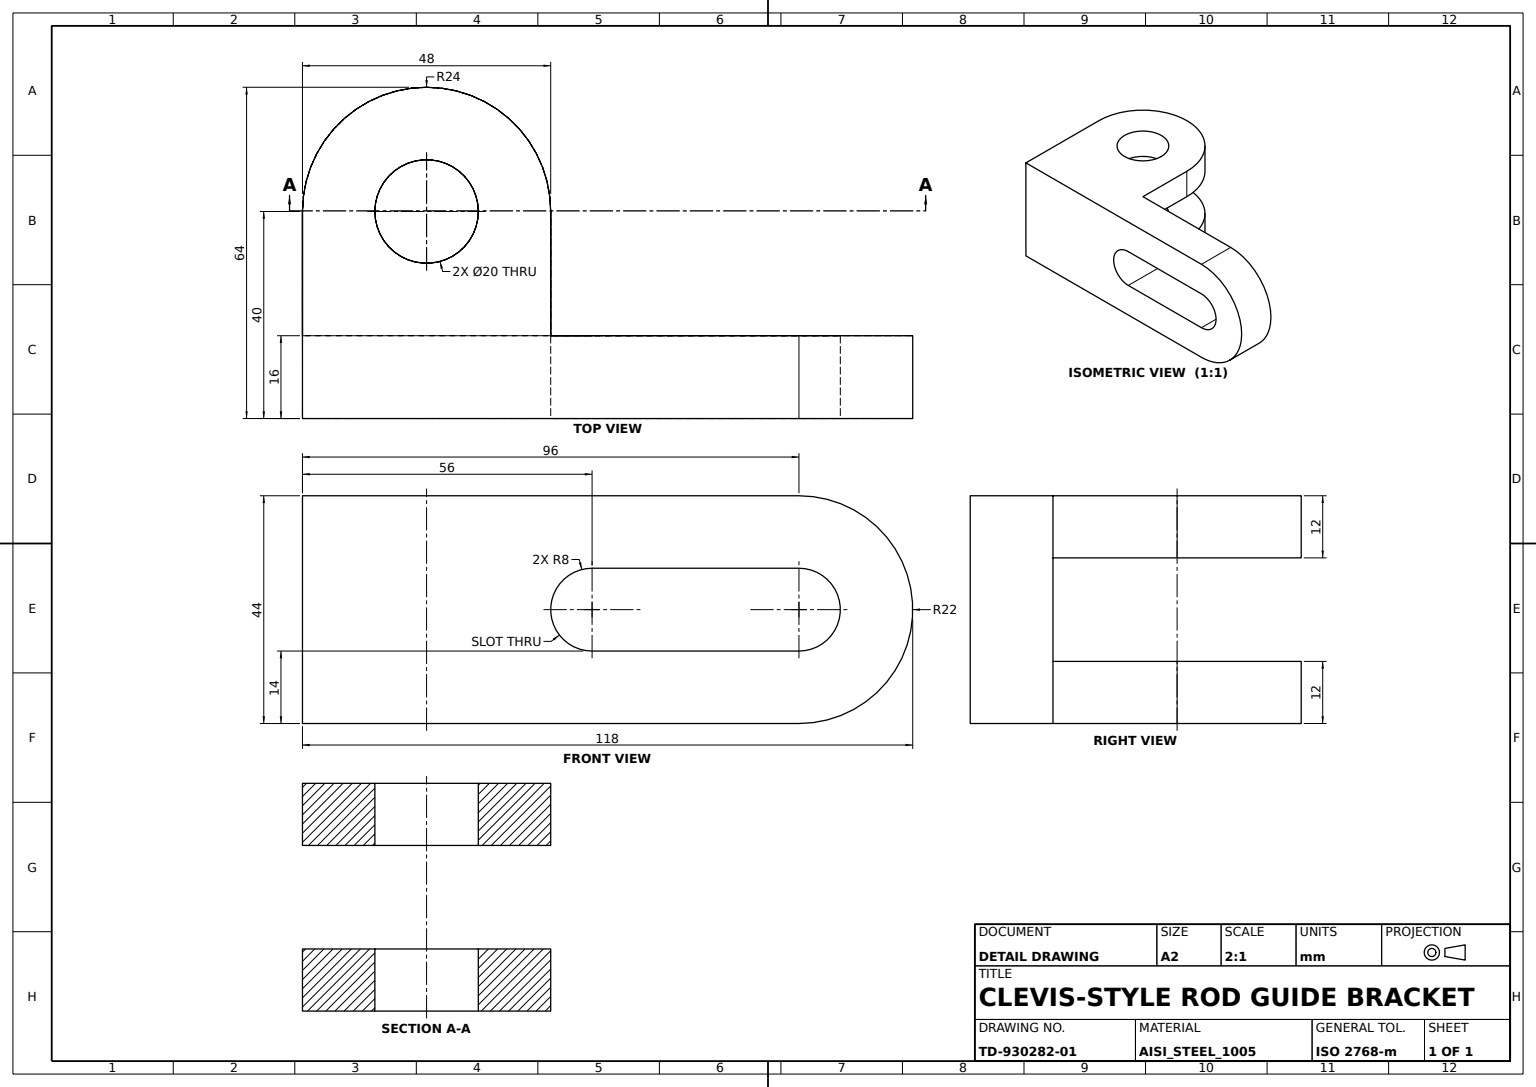
ISO-10303-21;
HEADER;
FILE_DESCRIPTION((''),'2;1');
FILE_NAME('','',(''),(''),'','','');
FILE_SCHEMA(('AUTOMOTIVE_DESIGN'));
ENDSEC;
DATA;
#1=APPLICATION_CONTEXT('');
#2=PRODUCT_CONTEXT('',#1,'mechanical');
#3=PRODUCT('','','',(#2));
#4=PRODUCT_DEFINITION_FORMATION('','',#3);
#5=PRODUCT_DEFINITION_CONTEXT('',#1,'design');
#6=PRODUCT_DEFINITION('','',#4,#5);
#7=PRODUCT_DEFINITION_SHAPE('','',#6);
#8=(LENGTH_UNIT()NAMED_UNIT(*)SI_UNIT(.MILLI.,.METRE.));
#9=(NAMED_UNIT(*)PLANE_ANGLE_UNIT()SI_UNIT($,.RADIAN.));
#10=(NAMED_UNIT(*)SI_UNIT($,.STERADIAN.)SOLID_ANGLE_UNIT());
#11=UNCERTAINTY_MEASURE_WITH_UNIT(LENGTH_MEASURE(0.005),#8,'distance_accuracy_value','');
#12=(GEOMETRIC_REPRESENTATION_CONTEXT(3)GLOBAL_UNCERTAINTY_ASSIGNED_CONTEXT((#11))GLOBAL_UNIT_ASSIGNED_CONTEXT((#8,#9,#10))REPRESENTATION_CONTEXT('',''));
#13=CARTESIAN_POINT('',(96.,16.,8.));
#14=VERTEX_POINT('',#13);
#15=CARTESIAN_POINT('',(96.,0.,8.));
#16=VERTEX_POINT('',#15);
#17=DIRECTION('',(0.,-1.,0.));
#18=VECTOR('',#17,1000.);
#19=LINE('',#13,#18);
#20=EDGE_CURVE('',#14,#16,#19,.T.);
#21=ORIENTED_EDGE('',*,*,#20,.F.);
#22=CARTESIAN_POINT('',(96.,16.,-8.));
#23=VERTEX_POINT('',#22);
#24=CARTESIAN_POINT('',(96.,16.,0.));
#25=DIRECTION('',(1.,0.,0.));
#26=AXIS2_PLACEMENT_3D('',#24,#17,#25);
#27=CIRCLE('',#26,8.);
#28=EDGE_CURVE('',#23,#14,#27,.T.);
#29=ORIENTED_EDGE('',*,*,#28,.F.);
#30=CARTESIAN_POINT('',(96.,0.,-8.));
#31=VERTEX_POINT('',#30);
#32=LINE('',#22,#18);
#33=EDGE_CURVE('',#23,#31,#32,.T.);
#34=ORIENTED_EDGE('',*,*,#33,.T.);
#35=CARTESIAN_POINT('',(96.,0.,0.));
#36=AXIS2_PLACEMENT_3D('',#35,#17,#25);
#37=CIRCLE('',#36,8.);
#38=EDGE_CURVE('',#31,#16,#37,.T.);
#39=ORIENTED_EDGE('',*,*,#38,.T.);
#40=EDGE_LOOP('',(#21,#29,#34,#39));
#41=FACE_BOUND('',#40,.T.);
#42=DIRECTION('',(0.,0.,-1.));
#43=AXIS2_PLACEMENT_3D('',#24,#17,#42);
#44=CYLINDRICAL_SURFACE('',#43,8.);
#45=ADVANCED_FACE('',(#41),#44,.F.);
#46=CARTESIAN_POINT('',(56.,16.,8.));
#47=VERTEX_POINT('',#46);
#48=DIRECTION('',(-1.,0.,0.));
#49=VECTOR('',#48,1000.);
#50=LINE('',#13,#49);
#51=EDGE_CURVE('',#14,#47,#50,.T.);
#52=ORIENTED_EDGE('',*,*,#51,.F.);
#53=ORIENTED_EDGE('',*,*,#20,.T.);
#54=CARTESIAN_POINT('',(56.,0.,8.));
#55=VERTEX_POINT('',#54);
#56=LINE('',#15,#49);
#57=EDGE_CURVE('',#16,#55,#56,.T.);
#58=ORIENTED_EDGE('',*,*,#57,.T.);
#59=LINE('',#46,#18);
#60=EDGE_CURVE('',#47,#55,#59,.T.);
#61=ORIENTED_EDGE('',*,*,#60,.F.);
#62=EDGE_LOOP('',(#52,#53,#58,#61));
#63=FACE_BOUND('',#62,.T.);
#64=DIRECTION('',(0.,0.,1.));
#65=AXIS2_PLACEMENT_3D('',#13,#64,#25);
#66=PLANE('',#65);
#67=ADVANCED_FACE('',(#63),#66,.F.);
#68=CARTESIAN_POINT('',(48.,40.,10.));
#69=VERTEX_POINT('',#68);
#70=CARTESIAN_POINT('',(48.,40.,22.));
#71=VERTEX_POINT('',#70);
#72=VECTOR('',#64,1000.);
#73=LINE('',#68,#72);
#74=EDGE_CURVE('',#69,#71,#73,.T.);
#75=ORIENTED_EDGE('',*,*,#74,.F.);
#76=CARTESIAN_POINT('',(0.,40.,10.));
#77=VERTEX_POINT('',#76);
#78=CARTESIAN_POINT('',(24.,40.,10.));
#79=AXIS2_PLACEMENT_3D('',#78,#64,#25);
#80=CIRCLE('',#79,24.);
#81=EDGE_CURVE('',#69,#77,#80,.T.);
#82=ORIENTED_EDGE('',*,*,#81,.T.);
#83=CARTESIAN_POINT('',(0.,40.,22.));
#84=VERTEX_POINT('',#83);
#85=LINE('',#76,#72);
#86=EDGE_CURVE('',#77,#84,#85,.T.);
#87=ORIENTED_EDGE('',*,*,#86,.T.);
#88=CARTESIAN_POINT('',(24.,40.,22.));
#89=AXIS2_PLACEMENT_3D('',#88,#64,#25);
#90=CIRCLE('',#89,24.);
#91=EDGE_CURVE('',#71,#84,#90,.T.);
#92=ORIENTED_EDGE('',*,*,#91,.F.);
#93=EDGE_LOOP('',(#75,#82,#87,#92));
#94=FACE_BOUND('',#93,.T.);
#95=CYLINDRICAL_SURFACE('',#79,24.);
#96=ADVANCED_FACE('',(#94),#95,.T.);
#97=ORIENTED_EDGE('',*,*,#60,.T.);
#98=CARTESIAN_POINT('',(56.,0.,-8.));
#99=VERTEX_POINT('',#98);
#100=CARTESIAN_POINT('',(56.,0.,0.));
#101=AXIS2_PLACEMENT_3D('',#100,#17,#25);
#102=CIRCLE('',#101,8.);
#103=EDGE_CURVE('',#55,#99,#102,.T.);
#104=ORIENTED_EDGE('',*,*,#103,.T.);
#105=CARTESIAN_POINT('',(56.,16.,-8.));
#106=VERTEX_POINT('',#105);
#107=LINE('',#105,#18);
#108=EDGE_CURVE('',#106,#99,#107,.T.);
#109=ORIENTED_EDGE('',*,*,#108,.F.);
#110=CARTESIAN_POINT('',(56.,16.,0.));
#111=AXIS2_PLACEMENT_3D('',#110,#17,#25);
#112=CIRCLE('',#111,8.);
#113=EDGE_CURVE('',#47,#106,#112,.T.);
#114=ORIENTED_EDGE('',*,*,#113,.F.);
#115=EDGE_LOOP('',(#97,#104,#109,#114));
#116=FACE_BOUND('',#115,.T.);
#117=AXIS2_PLACEMENT_3D('',#110,#17,#42);
#118=CYLINDRICAL_SURFACE('',#117,8.);
#119=ADVANCED_FACE('',(#116),#118,.F.);
#120=CARTESIAN_POINT('',(34.,40.,-22.));
#121=VERTEX_POINT('',#120);
#122=CARTESIAN_POINT('',(24.,40.,-22.));
#123=AXIS2_PLACEMENT_3D('',#122,#64,#25);
#124=CIRCLE('',#123,10.);
#125=EDGE_CURVE('',#121,#121,#124,.T.);
#126=ORIENTED_EDGE('',*,*,#125,.F.);
#127=EDGE_LOOP('',(#126));
#128=FACE_BOUND('',#127,.T.);
#129=CARTESIAN_POINT('',(34.,40.,-10.));
#130=VERTEX_POINT('',#129);
#131=CARTESIAN_POINT('',(24.,40.,-10.));
#132=AXIS2_PLACEMENT_3D('',#131,#64,#25);
#133=CIRCLE('',#132,10.);
#134=EDGE_CURVE('',#130,#130,#133,.T.);
#135=ORIENTED_EDGE('',*,*,#134,.T.);
#136=EDGE_LOOP('',(#135));
#137=FACE_BOUND('',#136,.T.);
#138=AXIS2_PLACEMENT_3D('',#131,#42,#48);
#139=CYLINDRICAL_SURFACE('',#138,10.);
#140=ADVANCED_FACE('',(#128,#137),#139,.F.);
#141=CARTESIAN_POINT('',(34.,40.,22.));
#142=VERTEX_POINT('',#141);
#143=CIRCLE('',#89,10.);
#144=EDGE_CURVE('',#142,#142,#143,.T.);
#145=ORIENTED_EDGE('',*,*,#144,.F.);
#146=EDGE_LOOP('',(#145));
#147=FACE_BOUND('',#146,.T.);
#148=CARTESIAN_POINT('',(48.,16.,22.));
#149=VERTEX_POINT('',#148);
#150=CARTESIAN_POINT('',(96.,16.,22.));
#151=VERTEX_POINT('',#150);
#152=CARTESIAN_POINT('',(0.,16.,22.));
#153=VECTOR('',#25,1000.);
#154=LINE('',#152,#153);
#155=EDGE_CURVE('',#149,#151,#154,.T.);
#156=ORIENTED_EDGE('',*,*,#155,.F.);
#157=DIRECTION('',(0.,1.,0.));
#158=VECTOR('',#157,1000.);
#159=LINE('',#148,#158);
#160=EDGE_CURVE('',#149,#71,#159,.T.);
#161=ORIENTED_EDGE('',*,*,#160,.T.);
#162=ORIENTED_EDGE('',*,*,#91,.T.);
#163=CARTESIAN_POINT('',(0.,0.,22.));
#164=VERTEX_POINT('',#163);
#165=LINE('',#152,#18);
#166=EDGE_CURVE('',#84,#164,#165,.T.);
#167=ORIENTED_EDGE('',*,*,#166,.T.);
#168=CARTESIAN_POINT('',(96.,0.,22.));
#169=VERTEX_POINT('',#168);
#170=LINE('',#163,#153);
#171=EDGE_CURVE('',#164,#169,#170,.T.);
#172=ORIENTED_EDGE('',*,*,#171,.T.);
#173=LINE('',#150,#18);
#174=EDGE_CURVE('',#151,#169,#173,.T.);
#175=ORIENTED_EDGE('',*,*,#174,.F.);
#176=EDGE_LOOP('',(#156,#161,#162,#167,#172,#175));
#177=FACE_BOUND('',#176,.T.);
#178=AXIS2_PLACEMENT_3D('',#152,#42,#48);
#179=PLANE('',#178);
#180=ADVANCED_FACE('',(#147,#177),#179,.F.);
#181=CARTESIAN_POINT('',(96.,0.,-22.));
#182=VERTEX_POINT('',#181);
#183=CARTESIAN_POINT('',(0.,0.,-22.));
#184=VERTEX_POINT('',#183);
#185=LINE('',#181,#49);
#186=EDGE_CURVE('',#182,#184,#185,.T.);
#187=ORIENTED_EDGE('',*,*,#186,.F.);
#188=AXIS2_PLACEMENT_3D('',#35,#157,#25);
#189=CIRCLE('',#188,22.);
#190=EDGE_CURVE('',#169,#182,#189,.T.);
#191=ORIENTED_EDGE('',*,*,#190,.F.);
#192=ORIENTED_EDGE('',*,*,#171,.F.);
#193=CARTESIAN_POINT('',(0.,0.,0.));
#194=LINE('',#193,#72);
#195=EDGE_CURVE('',#184,#164,#194,.T.);
#196=ORIENTED_EDGE('',*,*,#195,.F.);
#197=EDGE_LOOP('',(#187,#191,#192,#196));
#198=FACE_BOUND('',#197,.T.);
#199=LINE('',#98,#153);
#200=EDGE_CURVE('',#99,#31,#199,.T.);
#201=ORIENTED_EDGE('',*,*,#200,.F.);
#202=ORIENTED_EDGE('',*,*,#103,.F.);
#203=ORIENTED_EDGE('',*,*,#57,.F.);
#204=ORIENTED_EDGE('',*,*,#38,.F.);
#205=EDGE_LOOP('',(#201,#202,#203,#204));
#206=FACE_BOUND('',#205,.T.);
#207=AXIS2_PLACEMENT_3D('',#35,#157,#64);
#208=PLANE('',#207);
#209=ADVANCED_FACE('',(#198,#206),#208,.F.);
#210=ORIENTED_EDGE('',*,*,#190,.T.);
#211=CARTESIAN_POINT('',(96.,16.,-22.));
#212=VERTEX_POINT('',#211);
#213=LINE('',#211,#18);
#214=EDGE_CURVE('',#212,#182,#213,.T.);
#215=ORIENTED_EDGE('',*,*,#214,.F.);
#216=AXIS2_PLACEMENT_3D('',#24,#157,#25);
#217=CIRCLE('',#216,22.);
#218=EDGE_CURVE('',#151,#212,#217,.T.);
#219=ORIENTED_EDGE('',*,*,#218,.F.);
#220=ORIENTED_EDGE('',*,*,#174,.T.);
#221=EDGE_LOOP('',(#210,#215,#219,#220));
#222=FACE_BOUND('',#221,.T.);
#223=CYLINDRICAL_SURFACE('',#43,22.);
#224=ADVANCED_FACE('',(#222),#223,.T.);
#225=CARTESIAN_POINT('',(48.,16.,10.));
#226=VERTEX_POINT('',#225);
#227=LINE('',#225,#72);
#228=EDGE_CURVE('',#226,#149,#227,.T.);
#229=ORIENTED_EDGE('',*,*,#228,.T.);
#230=ORIENTED_EDGE('',*,*,#155,.T.);
#231=ORIENTED_EDGE('',*,*,#218,.T.);
#232=CARTESIAN_POINT('',(48.,16.,-22.));
#233=VERTEX_POINT('',#232);
#234=LINE('',#211,#49);
#235=EDGE_CURVE('',#212,#233,#234,.T.);
#236=ORIENTED_EDGE('',*,*,#235,.T.);
#237=CARTESIAN_POINT('',(48.,16.,-10.));
#238=VERTEX_POINT('',#237);
#239=VECTOR('',#42,1000.);
#240=LINE('',#237,#239);
#241=EDGE_CURVE('',#238,#233,#240,.T.);
#242=ORIENTED_EDGE('',*,*,#241,.F.);
#243=CARTESIAN_POINT('',(0.,16.,-10.));
#244=VERTEX_POINT('',#243);
#245=LINE('',#243,#153);
#246=EDGE_CURVE('',#244,#238,#245,.T.);
#247=ORIENTED_EDGE('',*,*,#246,.F.);
#248=CARTESIAN_POINT('',(0.,16.,10.));
#249=VERTEX_POINT('',#248);
#250=CARTESIAN_POINT('',(0.,16.,-22.));
#251=LINE('',#250,#72);
#252=EDGE_CURVE('',#244,#249,#251,.T.);
#253=ORIENTED_EDGE('',*,*,#252,.T.);
#254=LINE('',#248,#153);
#255=EDGE_CURVE('',#249,#226,#254,.T.);
#256=ORIENTED_EDGE('',*,*,#255,.T.);
#257=EDGE_LOOP('',(#229,#230,#231,#236,#242,#247,#253,#256));
#258=FACE_BOUND('',#257,.T.);
#259=ORIENTED_EDGE('',*,*,#113,.T.);
#260=LINE('',#105,#153);
#261=EDGE_CURVE('',#106,#23,#260,.T.);
#262=ORIENTED_EDGE('',*,*,#261,.T.);
#263=ORIENTED_EDGE('',*,*,#28,.T.);
#264=ORIENTED_EDGE('',*,*,#51,.T.);
#265=EDGE_LOOP('',(#259,#262,#263,#264));
#266=FACE_BOUND('',#265,.T.);
#267=AXIS2_PLACEMENT_3D('',#24,#157,#64);
#268=PLANE('',#267);
#269=ADVANCED_FACE('',(#258,#266),#268,.T.);
#270=ORIENTED_EDGE('',*,*,#144,.T.);
#271=EDGE_LOOP('',(#270));
#272=FACE_BOUND('',#271,.T.);
#273=CARTESIAN_POINT('',(34.,40.,10.));
#274=VERTEX_POINT('',#273);
#275=CIRCLE('',#79,10.);
#276=EDGE_CURVE('',#274,#274,#275,.T.);
#277=ORIENTED_EDGE('',*,*,#276,.F.);
#278=EDGE_LOOP('',(#277));
#279=FACE_BOUND('',#278,.T.);
#280=CYLINDRICAL_SURFACE('',#79,10.);
#281=ADVANCED_FACE('',(#272,#279),#280,.F.);
#282=ORIENTED_EDGE('',*,*,#86,.F.);
#283=LINE('',#76,#18);
#284=EDGE_CURVE('',#77,#249,#283,.T.);
#285=ORIENTED_EDGE('',*,*,#284,.T.);
#286=ORIENTED_EDGE('',*,*,#252,.F.);
#287=CARTESIAN_POINT('',(0.,40.,-10.));
#288=VERTEX_POINT('',#287);
#289=LINE('',#287,#18);
#290=EDGE_CURVE('',#288,#244,#289,.T.);
#291=ORIENTED_EDGE('',*,*,#290,.F.);
#292=CARTESIAN_POINT('',(0.,40.,-22.));
#293=VERTEX_POINT('',#292);
#294=LINE('',#287,#239);
#295=EDGE_CURVE('',#288,#293,#294,.T.);
#296=ORIENTED_EDGE('',*,*,#295,.T.);
#297=LINE('',#250,#18);
#298=EDGE_CURVE('',#293,#184,#297,.T.);
#299=ORIENTED_EDGE('',*,*,#298,.T.);
#300=ORIENTED_EDGE('',*,*,#195,.T.);
#301=ORIENTED_EDGE('',*,*,#166,.F.);
#302=EDGE_LOOP('',(#282,#285,#286,#291,#296,#299,#300,#301));
#303=FACE_BOUND('',#302,.T.);
#304=CARTESIAN_POINT('',(0.,16.,0.));
#305=AXIS2_PLACEMENT_3D('',#304,#25,#42);
#306=PLANE('',#305);
#307=ADVANCED_FACE('',(#303),#306,.F.);
#308=ORIENTED_EDGE('',*,*,#160,.F.);
#309=ORIENTED_EDGE('',*,*,#228,.F.);
#310=LINE('',#225,#158);
#311=EDGE_CURVE('',#226,#69,#310,.T.);
#312=ORIENTED_EDGE('',*,*,#311,.T.);
#313=ORIENTED_EDGE('',*,*,#74,.T.);
#314=EDGE_LOOP('',(#308,#309,#312,#313));
#315=FACE_BOUND('',#314,.T.);
#316=AXIS2_PLACEMENT_3D('',#225,#25,#157);
#317=PLANE('',#316);
#318=ADVANCED_FACE('',(#315),#317,.T.);
#319=ORIENTED_EDGE('',*,*,#255,.F.);
#320=ORIENTED_EDGE('',*,*,#284,.F.);
#321=ORIENTED_EDGE('',*,*,#81,.F.);
#322=ORIENTED_EDGE('',*,*,#311,.F.);
#323=EDGE_LOOP('',(#319,#320,#321,#322));
#324=FACE_BOUND('',#323,.T.);
#325=ORIENTED_EDGE('',*,*,#276,.T.);
#326=EDGE_LOOP('',(#325));
#327=FACE_BOUND('',#326,.T.);
#328=PLANE('',#79);
#329=ADVANCED_FACE('',(#324,#327),#328,.F.);
#330=ORIENTED_EDGE('',*,*,#33,.F.);
#331=ORIENTED_EDGE('',*,*,#261,.F.);
#332=ORIENTED_EDGE('',*,*,#108,.T.);
#333=ORIENTED_EDGE('',*,*,#200,.T.);
#334=EDGE_LOOP('',(#330,#331,#332,#333));
#335=FACE_BOUND('',#334,.T.);
#336=AXIS2_PLACEMENT_3D('',#105,#42,#48);
#337=PLANE('',#336);
#338=ADVANCED_FACE('',(#335),#337,.F.);
#339=CARTESIAN_POINT('',(48.,40.,-22.));
#340=VERTEX_POINT('',#339);
#341=LINE('',#232,#158);
#342=EDGE_CURVE('',#233,#340,#341,.T.);
#343=ORIENTED_EDGE('',*,*,#342,.T.);
#344=CARTESIAN_POINT('',(48.,40.,-10.));
#345=VERTEX_POINT('',#344);
#346=LINE('',#344,#239);
#347=EDGE_CURVE('',#345,#340,#346,.T.);
#348=ORIENTED_EDGE('',*,*,#347,.F.);
#349=LINE('',#237,#158);
#350=EDGE_CURVE('',#238,#345,#349,.T.);
#351=ORIENTED_EDGE('',*,*,#350,.F.);
#352=ORIENTED_EDGE('',*,*,#241,.T.);
#353=EDGE_LOOP('',(#343,#348,#351,#352));
#354=FACE_BOUND('',#353,.T.);
#355=AXIS2_PLACEMENT_3D('',#237,#48,#17);
#356=PLANE('',#355);
#357=ADVANCED_FACE('',(#354),#356,.F.);
#358=CIRCLE('',#132,24.);
#359=EDGE_CURVE('',#345,#288,#358,.T.);
#360=ORIENTED_EDGE('',*,*,#359,.F.);
#361=ORIENTED_EDGE('',*,*,#347,.T.);
#362=CIRCLE('',#123,24.);
#363=EDGE_CURVE('',#340,#293,#362,.T.);
#364=ORIENTED_EDGE('',*,*,#363,.T.);
#365=ORIENTED_EDGE('',*,*,#295,.F.);
#366=EDGE_LOOP('',(#360,#361,#364,#365));
#367=FACE_BOUND('',#366,.T.);
#368=CYLINDRICAL_SURFACE('',#138,24.);
#369=ADVANCED_FACE('',(#367),#368,.T.);
#370=ORIENTED_EDGE('',*,*,#134,.F.);
#371=EDGE_LOOP('',(#370));
#372=FACE_BOUND('',#371,.T.);
#373=ORIENTED_EDGE('',*,*,#290,.T.);
#374=ORIENTED_EDGE('',*,*,#246,.T.);
#375=ORIENTED_EDGE('',*,*,#350,.T.);
#376=ORIENTED_EDGE('',*,*,#359,.T.);
#377=EDGE_LOOP('',(#373,#374,#375,#376));
#378=FACE_BOUND('',#377,.T.);
#379=PLANE('',#132);
#380=ADVANCED_FACE('',(#372,#378),#379,.T.);
#381=ORIENTED_EDGE('',*,*,#125,.T.);
#382=EDGE_LOOP('',(#381));
#383=FACE_BOUND('',#382,.T.);
#384=ORIENTED_EDGE('',*,*,#342,.F.);
#385=ORIENTED_EDGE('',*,*,#235,.F.);
#386=ORIENTED_EDGE('',*,*,#214,.T.);
#387=ORIENTED_EDGE('',*,*,#186,.T.);
#388=ORIENTED_EDGE('',*,*,#298,.F.);
#389=ORIENTED_EDGE('',*,*,#363,.F.);
#390=EDGE_LOOP('',(#384,#385,#386,#387,#388,#389));
#391=FACE_BOUND('',#390,.T.);
#392=AXIS2_PLACEMENT_3D('',#211,#64,#25);
#393=PLANE('',#392);
#394=ADVANCED_FACE('',(#383,#391),#393,.F.);
#395=CLOSED_SHELL('',(#45,#67,#96,#119,#140,#180,#209,#224,#269,#281,#307,#318,#329,#338,#357,#369,#380,#394));
#396=MANIFOLD_SOLID_BREP('',#395);
#397=ADVANCED_BREP_SHAPE_REPRESENTATION('',(#396),#12);
#398=SHAPE_DEFINITION_REPRESENTATION(#7,#397);
ENDSEC;
END-ISO-10303-21;
